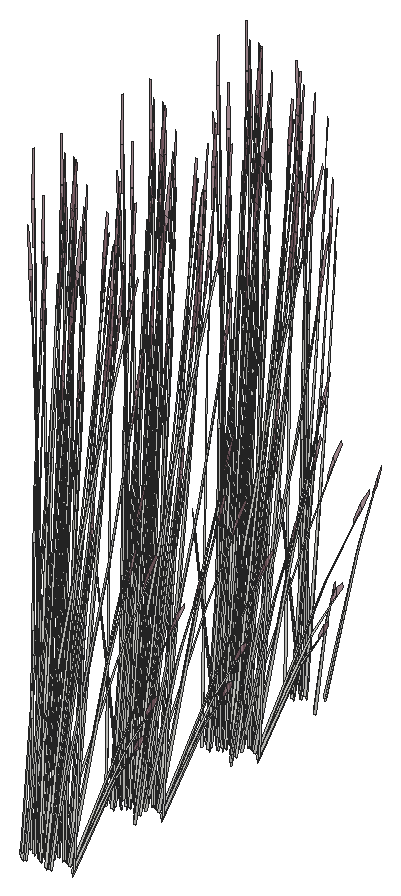
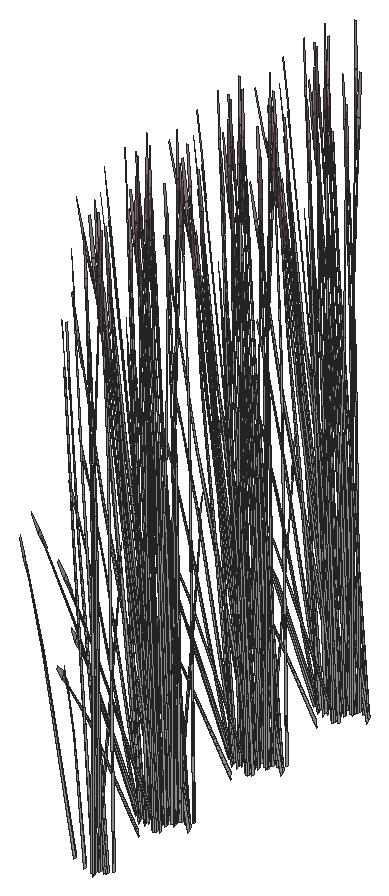
# SketchUp Ruby script. Lengths in inches.
U = 1.inch
M = Sketchup.active_model
def pt(a) = Geom::Point3d.new(a.map { |v| v * U })
def face(e, loops, mat)
  f = e.add_face(loops[0].map { |a| pt(a) })
  loops[1..].each { |l| e.add_face(l.map { |a| pt(a) }).erase! }
  f.material = f.back_material = mat if mat
  f
end
# faces: each face lists its corners as indices into pts; further lists are holes
def faces(e, pts, list, mat = nil) = list.each { |f| face(e, (f[0].is_a?(Array) ? f : [f]).map { |l| l.map { |i| pts[i] } }, mat) }
# xy, xz, yz: faces in a plane at the given z, y or x. An outline is a flat list of corners, or four numbers for a rectangle; further outlines are holes
def ring(l) = l.size == 4 ? [[l[0], l[1]], [l[2], l[1]], [l[2], l[3]], [l[0], l[3]]] : l.each_slice(2).to_a
def flat(e, list, mat, &to3) = list.each { |f| face(e, (f[0].is_a?(Array) ? f : [f]).map { |l| ring(l).map { |u, v| to3.(u, v) } }, mat) }
def xy(e, z, list, mat = nil) = flat(e, list, mat) { |x, y| [x, y, z] }
def xz(e, y, list, mat = nil) = flat(e, list, mat) { |x, z| [x, y, z] }
def yz(e, x, list, mat = nil) = flat(e, list, mat) { |y, z| [x, y, z] }
def lines(e, pts, list) = list.each { |a, b| e.add_line(pt(pts[a]), pt(pts[b])) }
# prism: a flat outline (further loops are holes) pulled along v
def prism(e, loops, v, mat = nil)
  f = face(e, loops, mat); d = Geom::Vector3d.new(v.map { |x| x * U })
  f.pushpull(f.normal.samedirection?(d) ? d.length : -d.length)
end
def box(e, o, s, mat = nil) = prism(e, [[o, [o[0] + s[0], o[1], o[2]], [o[0] + s[0], o[1] + s[1], o[2]], [o[0], o[1] + s[1], o[2]]]], [0, 0, s[2]], mat)
def at(x, y, z, deg = 0) = Geom::Transformation.translation(pt([x, y, z])) * Geom::Transformation.rotation(ORIGIN, Z_AXIS, deg.degrees)
def axes(o, x, y, z) = Geom::Transformation.new([*x, 0, *y, 0, *z, 0, *pt(o).to_a, 1])
def part(name) = M.definitions.add(name)
# library, detail: a bought-in or finely detailed component or shape, given as its bounding box
def library(name, o, s) = part(name).tap { |d| box(d.entities, o, s) }
def detail(e, o, s) = box(e.add_group.entities, o, s)
def put(e, d, t, mat = nil) = e.add_instance(d, t).tap { |i| i.material = mat if mat }
def group(e, t, mat = nil) = e.add_group.tap { |g| g.transformation = t; g.material = mat if mat }.entities
root = M.entities
M.materials.add("LightPink_Translucent").color = [144, 107, 117]
M.materials["LightPink_Translucent"].alpha = 0.75
c1 = part("blade")
p = [[2.15,0.21,22],[0,0.17,0],[0.09,0.45,0],[2.18,0.31,22],[2.29,0.31,22],[0.38,0.45,0],
  [2.48,0.24,33],[2.49,0.24,33],[2.48,0.22,33]]
faces(c1.entities,p,[[0,1,2,3],[4,5,2,3],[6,3,4,7],[8,0,3,6]])
c2 = part("seeds")
p = [[0.3,-0.1,1.38],[-0.01,-0.03,1.59],[-0.01,-0.03,0.03],[0.14,-0.07,-0.07],[0.29,-0.03,3],[0.15,0.01,3.11]]
faces(c2.entities,p,[[0,1,2,3],[1,0,4,5]],"LightPink_Translucent")
c3 = part("blade with seeds")
put(c3.entities,c1,at(0,0,0))
put(c3.entities,c2,axes([2.4,0.25,30.99],[1.5799,-0.05474,1.17369],[-0.12525,1.92788,0.29478],[-0.07173,-0.02425,1.56792]))
put(root,c3,axes([333.54,335.91,50.36],[-0.05884,-0.44587,-0.25709],[0.6128,-0.02696,-0.44182],[0.10791,-0.05939,1.41118]))
put(root,c3,axes([333.46,334.92,49.79],[0.47106,0.09668,-0.27372],[-0.11861,0.34048,0.27372],[0.09497,-0.03926,1.22797]))
put(root,c3,axes([333.62,336.26,50.15],[0.56891,0.18939,0.21263],[-0.2738,0.39352,0.44182],[0,-0.09071,1.41855]))
put(root,c3,axes([333.44,335.99,50.4],[-0.54829,0.02412,0.39531],[-0.04958,-0.40041,-0.19025],[0.09816,-0.04058,1.26923]))
put(root,c3,axes([335.24,334.92,50.1],[0.31568,-0.39156,0],[0.52815,0.21836,-0.456],[0.12029,0.04973,1.44655]))
put(root,c3,axes([336.49,336.47,49.75],[-0.3252,0.04689,1.25103],[-0.05176,-0.37326,0.07161],[0.22777,-0.0565,0.71188]))
put(root,c3,axes([337.08,336.14,50],[-0.31304,-0.24986,-0.05733],[0.34284,-0.22894,-0.25992],[0.09714,-0.01612,0.85731]))
put(root,c3,axes([334.21,336.17,49.95],[0,-0.45213,0],[0.63136,0,0],[0,0,1.58567]))
put(root,c3,axes([334.97,335.13,50.19],[-0.47255,-0.19538,0.43871],[0.28245,-0.35034,0],[0.10763,0.0445,1.3917]))
put(root,c3,axes([333.91,335.89,50.09],[-0.41865,0.35461,0.40429],[-0.49737,-0.31303,0.15865],[0.10093,-0.03539,1.40366]))
put(root,c3,axes([333.18,335.31,50.1875],[-0.14586,0.38834,0.15589],[-0.53375,-0.1099,0.31002],[0.0922,-0.00189,1.41735]))
put(root,c3,axes([332.96,335.62,49.41],[-0.49699,0.15644,1.13921],[-0.15819,-0.44887,0.44265],[0.30518,0.00747,1.29573]))
put(root,c3,axes([334.29,335.74,50.3125],[0.09741,-0.34873,0.12794],[0.4759,0.06053,-0.36534],[0.08661,0.03581,1.11991]))
put(root,c3,axes([336.84,336.23,49.32],[-0.02639,-0.05932,1.55816],[0.18302,-0.34702,-0.23804],[0.18462,-0.00499,0.26541]))
put(root,c3,axes([334.09,335.83,50.4],[-0.30332,-0.32798,0.39531],[0.45944,-0.23096,-0.19025],[0.09816,0.04058,1.26923]))
put(root,c3,axes([334.25,335.85,50.36],[0.50979,-0.25942,-0.25709],[0.339,0.36656,-0.44182],[0.12578,0.03723,1.41118]))
put(root,c3,axes([335.53,335.16,49.78],[0.47255,0.19538,-0.43871],[-0.28245,0.35034,0],[0.10763,0.0445,1.3917]))
put(root,c3,axes([334.63,336.28,49.95],[0.56491,0,0],[0,0.40454,0],[0,0,1.5764]))
put(root,c3,axes([334.79,335.33,50.1875],[-0.54257,0.10371,0.15589],[-0.13397,-0.38597,0.31002],[0.04839,0.05624,1.41735]))
put(root,c3,axes([335.4,335.31,49.79],[0.11861,0.34048,-0.27372],[-0.47106,0.09668,0.27372],[0.09497,0.03926,1.22797]))
put(root,c3,axes([334.45,336.07,50.1],[-0.63817,-0.08233,0.43472],[0.12987,-0.46497,0.17059],[0.09326,0.0449,1.50931]))
put(root,c3,axes([334.56,337.17,49.93],[0.53009,-0.13258,-0.16963],[0.18627,0.38191,0.00007],[0.05851,-0.01465,1.53656]))
put(root,c3,axes([334.62,336.45,49.96],[0.35245,0.2524,0],[-0.35245,0.2524,0],[0,0,1.49564]))
put(root,c3,axes([335.58,336.34,50.1875],[-0.39671,-0.28463,0.15589],[0.39978,-0.27607,0.31002],[-0.04381,0.05813,1.41735]))
put(root,c3,axes([334.84,335.91,49.82],[0.52523,0.06406,-0.55095],[-0.11084,0.39517,-0.1446],[0.15674,0.04788,1.21613]))
put(root,c3,axes([334.62,336.15,50.4],[0.24498,-0.3521,0.39531],[0.50902,0.16945,-0.19025],[0,0.08116,1.26923]))
put(root,c3,axes([334.52,336.35,50.03],[0,0.45191,-0.04981],[-0.63136,0,0],[0,0.0142,1.58489]))
put(root,c3,axes([334.57,336.03,49.95],[0.30332,0.32798,-0.39531],[-0.45944,0.23096,0.19025],[0.09816,0.04058,1.26923]))
put(root,c3,axes([335.9,336.35,50.19],[0,-0.39075,0.43871],[0.56491,0,0],[0,0.089,1.3917]))
put(root,c3,axes([334.83,336.23,50.3125],[0.47043,-0.11396,0.12794],[0.16474,0.32541,-0.36534],[0,0.07162,1.11991]))
put(root,c3,axes([336.58,337.03,50.29],[-0.1216,-0.0961,1.26356],[0.15822,-0.31792,-0.27174],[0.24603,0.04307,0.54024]))
put(root,c3,axes([334.4,337.375,49.95],[0.50902,0.17543,0],[-0.24498,0.36452,0],[0,0,1.54589]))
put(root,c3,axes([334.22,337.23,50.02],[0.21952,0.44891,-0.05313],[-0.62724,0.1573,0],[0.00767,0.01568,1.52132]))
put(root,c3,axes([336.29,336.42,50.1],[0.63136,0,0],[0,0.43672,-0.456],[0,0.09947,1.44655]))
put(root,c3,axes([336.03,336.64,49.94],[-0.63105,-0.00312,-0.04397],[0,-0.43672,0.44129],[-0.01983,0.09942,1.3992]))
put(root,c3,axes([334.67,336.26,50.36],[0.56863,0.18645,-0.25709],[-0.2738,0.39352,-0.44182],[0.01787,0.09662,1.41118]))
put(root,c3,axes([335.9,336.7,49.79],[-0.35245,0.2438,-0.27372],[-0.35245,-0.2438,0.27372],[0,0.07853,1.22797]))
put(root,c3,axes([336.15,336.71,49.78],[0,0.39075,-0.43871],[-0.56491,0,0],[0,0.089,1.3917]))
put(root,c3,axes([335.51,337.94,49.32],[0.03679,-0.05641,1.55816],[0.46313,-0.16615,-0.23804],[0.14041,0.08599,0.26541]))
put(root,c3,axes([334.9,336.66,49.85],[0.18514,0.35777,-0.61156],[-0.53331,0.12885,-0.16051],[0.02046,0.12115,1.3499]))
put(root,c3,axes([335.47,338.03,50.36],[-0.32378,-0.01225,0.92831],[0.21383,-0.26028,0.51254],[0.12791,0.09247,0.72818]))
put(root,c3,axes([334.42,337.4,50.29],[0.00891,-0.12953,1.26356],[0.4258,-0.14469,-0.27174],[0.13144,0.15503,0.54024]))
put(root,c3,axes([334.77,344.44,50.29],[-0.14352,0.07909,1.26356],[-0.42983,-0.13843,-0.27174],[0.07968,-0.17216,0.54024]))
put(root,c3,axes([335.77,344.6875,49.32],[-0.07557,-0.03078,1.55816],[-0.19412,-0.34391,-0.23804],[0.13095,-0.09333,0.26541]))
put(root,c3,axes([332.92,344.76,50.1],[-0.31568,-0.39156,0],[0.52815,-0.21836,-0.456],[0.12029,-0.04973,1.44655]))
put(root,c3,axes([333.35,344.7,49.78],[0.47255,-0.19538,-0.43871],[0.28245,0.35034,0],[0.10763,-0.0445,1.3917]))
put(root,c3,axes([336.15,345.375,50.29],[-0.18038,-0.01157,1.26356],[-0.18479,-0.31048,-0.27174],[0.22159,-0.08783,0.54024]))
put(root,c3,axes([333.91,345.5,49.82],[0.34009,-0.2937,-0.55095],[0.42248,0.26632,-0.1446],[0.13628,-0.07327,1.21613]))
put(root,c3,axes([333.54,345.84,50.36],[-0.05884,-0.44587,-0.25709],[0.6128,-0.02696,-0.44182],[0.10791,-0.05939,1.41118]))
put(root,c3,axes([333.46,344.86,49.79],[0.47106,0.09668,-0.27372],[-0.11861,0.34048,0.27372],[0.09497,-0.03926,1.22797]))
put(root,c3,axes([333.62,346.19,50.15],[0.56891,0.18939,0.21263],[-0.2738,0.39352,0.44182],[0,-0.09071,1.41855]))
put(root,c3,axes([333.44,345.93,50.4],[-0.54829,0.02412,0.39531],[-0.04958,-0.40041,-0.19025],[0.09816,-0.04058,1.26923]))
put(root,c3,axes([335.24,344.86,50.1],[0.31568,-0.39156,0],[0.52815,0.21836,-0.456],[0.12029,0.04973,1.44655]))
put(root,c3,axes([336.49,346.41,49.75],[-0.3252,0.04689,1.25103],[-0.05176,-0.37326,0.07161],[0.22777,-0.0565,0.71188]))
put(root,c3,axes([337.08,346.08,50],[-0.31304,-0.24986,-0.05733],[0.34284,-0.22894,-0.25992],[0.09714,-0.01612,0.85731]))
put(root,c3,axes([334.21,346.11,49.95],[0,-0.45213,0],[0.63136,0,0],[0,0,1.58567]))
put(root,c3,axes([334.97,345.06,50.19],[-0.47255,-0.19538,0.43871],[0.28245,-0.35034,0],[0.10763,0.0445,1.3917]))
put(root,c3,axes([333.91,345.82,50.09],[-0.41865,0.35461,0.40429],[-0.49737,-0.31303,0.15865],[0.10093,-0.03539,1.40366]))
put(root,c3,axes([333.18,345.24,50.1875],[-0.14586,0.38834,0.15589],[-0.53375,-0.1099,0.31002],[0.0922,-0.00189,1.41735]))
put(root,c3,axes([332.96,345.55,49.41],[-0.49699,0.15644,1.13921],[-0.15819,-0.44887,0.44265],[0.30518,0.00747,1.29573]))
put(root,c3,axes([334.29,345.67,50.3125],[0.09741,-0.34873,0.12794],[0.4759,0.06053,-0.36534],[0.08661,0.03581,1.11991]))
put(root,c3,axes([336.84,346.16,49.32],[-0.02639,-0.05932,1.55816],[0.18302,-0.34702,-0.23804],[0.18462,-0.00499,0.26541]))
put(root,c3,axes([334.09,345.76,50.4],[-0.30332,-0.32798,0.39531],[0.45944,-0.23096,-0.19025],[0.09816,0.04058,1.26923]))
put(root,c3,axes([334.25,345.79,50.36],[0.50979,-0.25942,-0.25709],[0.339,0.36656,-0.44182],[0.12578,0.03723,1.41118]))
put(root,c3,axes([335.53,345.1,49.78],[0.47255,0.19538,-0.43871],[-0.28245,0.35034,0],[0.10763,0.0445,1.3917]))
put(root,c3,axes([334.63,346.21,49.95],[0.56491,0,0],[0,0.40454,0],[0,0,1.5764]))
put(root,c3,axes([334.79,345.26,50.1875],[-0.54257,0.10371,0.15589],[-0.13397,-0.38597,0.31002],[0.04839,0.05624,1.41735]))
put(root,c3,axes([335.4,345.24,49.79],[0.11861,0.34048,-0.27372],[-0.47106,0.09668,0.27372],[0.09497,0.03926,1.22797]))
put(root,c3,axes([334.45,346,50.1],[-0.63817,-0.08233,0.43472],[0.12987,-0.46497,0.17059],[0.09326,0.0449,1.50931]))
put(root,c3,axes([334.56,347.11,49.93],[0.53009,-0.13258,-0.16963],[0.18627,0.38191,0.00007],[0.05851,-0.01465,1.53656]))
put(root,c3,axes([334.62,346.38,49.96],[0.35245,0.2524,0],[-0.35245,0.2524,0],[0,0,1.49564]))
put(root,c3,axes([335.58,346.27,50.1875],[-0.39671,-0.28463,0.15589],[0.39978,-0.27607,0.31002],[-0.04381,0.05813,1.41735]))
put(root,c3,axes([334.84,345.84,49.82],[0.52523,0.06406,-0.55095],[-0.11084,0.39517,-0.1446],[0.15674,0.04788,1.21613]))
put(root,c3,axes([334.62,346.09,50.4],[0.24498,-0.3521,0.39531],[0.50902,0.16945,-0.19025],[0,0.08116,1.26923]))
put(root,c3,axes([334.52,346.29,50.03],[0,0.45191,-0.04981],[-0.63136,0,0],[0,0.0142,1.58489]))
put(root,c3,axes([334.57,345.97,49.95],[0.30332,0.32798,-0.39531],[-0.45944,0.23096,0.19025],[0.09816,0.04058,1.26923]))
put(root,c3,axes([335.9,346.28,50.19],[0,-0.39075,0.43871],[0.56491,0,0],[0,0.089,1.3917]))
put(root,c3,axes([334.83,346.17,50.3125],[0.47043,-0.11396,0.12794],[0.16474,0.32541,-0.36534],[0,0.07162,1.11991]))
put(root,c3,axes([336.58,346.96,50.29],[-0.1216,-0.0961,1.26356],[0.15822,-0.31792,-0.27174],[0.24603,0.04307,0.54024]))
put(root,c3,axes([334.4,347.3125,49.95],[0.50902,0.17543,0],[-0.24498,0.36452,0],[0,0,1.54589]))
put(root,c3,axes([334.22,347.16,50.02],[0.21952,0.44891,-0.05313],[-0.62724,0.1573,0],[0.00767,0.01568,1.52132]))
put(root,c3,axes([336.29,346.35,50.1],[0.63136,0,0],[0,0.43672,-0.456],[0,0.09947,1.44655]))
put(root,c3,axes([336.03,346.58,49.94],[-0.63105,-0.00312,-0.04397],[0,-0.43672,0.44129],[-0.01983,0.09942,1.3992]))
put(root,c3,axes([334.67,346.2,50.36],[0.56863,0.18645,-0.25709],[-0.2738,0.39352,-0.44182],[0.01787,0.09662,1.41118]))
put(root,c3,axes([335.9,346.64,49.79],[-0.35245,0.2438,-0.27372],[-0.35245,-0.2438,0.27372],[0,0.07853,1.22797]))
put(root,c3,axes([336.15,346.65,49.78],[0,0.39075,-0.43871],[-0.56491,0,0],[0,0.089,1.3917]))
put(root,c3,axes([335.51,347.875,49.32],[0.03679,-0.05641,1.55816],[0.46313,-0.16615,-0.23804],[0.14041,0.08599,0.26541]))
put(root,c3,axes([334.9,346.59,49.85],[0.18514,0.35777,-0.61156],[-0.53331,0.12885,-0.16051],[0.02046,0.12115,1.3499]))
put(root,c3,axes([335.47,347.97,50.36],[-0.32378,-0.01225,0.92831],[0.21383,-0.26028,0.51254],[0.12791,0.09247,0.72818]))
put(root,c3,axes([334.42,347.34,50.29],[0.00891,-0.12953,1.26356],[0.4258,-0.14469,-0.27174],[0.13144,0.15503,0.54024]))
put(root,c3,axes([334.77,355.17,50.29],[-0.14352,0.07909,1.26356],[-0.42983,-0.13843,-0.27174],[0.07968,-0.17216,0.54024]))
put(root,c3,axes([335.77,355.41,49.32],[-0.07557,-0.03078,1.55816],[-0.19412,-0.34391,-0.23804],[0.13095,-0.09333,0.26541]))
put(root,c3,axes([332.92,355.48,50.1],[-0.31568,-0.39156,0],[0.52815,-0.21836,-0.456],[0.12029,-0.04973,1.44655]))
put(root,c3,axes([333.35,355.42,49.78],[0.47255,-0.19538,-0.43871],[0.28245,0.35034,0],[0.10763,-0.0445,1.3917]))
put(root,c3,axes([336.15,356.1,50.29],[-0.18038,-0.01157,1.26356],[-0.18479,-0.31048,-0.27174],[0.22159,-0.08783,0.54024]))
put(root,c3,axes([333.91,356.22,49.82],[0.34009,-0.2937,-0.55095],[0.42248,0.26632,-0.1446],[0.13628,-0.07327,1.21613]))
put(root,c3,axes([333.54,356.56,50.36],[-0.05884,-0.44587,-0.25709],[0.6128,-0.02696,-0.44182],[0.10791,-0.05939,1.41118]))
put(root,c3,axes([333.46,355.58,49.79],[0.47106,0.09668,-0.27372],[-0.11861,0.34048,0.27372],[0.09497,-0.03926,1.22797]))
put(root,c3,axes([333.62,356.91,50.15],[0.56891,0.18939,0.21263],[-0.2738,0.39352,0.44182],[0,-0.09071,1.41855]))
put(root,c3,axes([333.44,356.65,50.4],[-0.54829,0.02412,0.39531],[-0.04958,-0.40041,-0.19025],[0.09816,-0.04058,1.26923]))
put(root,c3,axes([335.24,355.58,50.1],[0.31568,-0.39156,0],[0.52815,0.21836,-0.456],[0.12029,0.04973,1.44655]))
put(root,c3,axes([336.49,357.13,49.75],[-0.3252,0.04689,1.25103],[-0.05176,-0.37326,0.07161],[0.22777,-0.0565,0.71188]))
put(root,c3,axes([337.08,356.8,50],[-0.31304,-0.24986,-0.05733],[0.34284,-0.22894,-0.25992],[0.09714,-0.01612,0.85731]))
put(root,c3,axes([334.21,356.83,49.95],[0,-0.45213,0],[0.63136,0,0],[0,0,1.58567]))
put(root,c3,axes([334.97,355.79,50.19],[-0.47255,-0.19538,0.43871],[0.28245,-0.35034,0],[0.10763,0.0445,1.3917]))
put(root,c3,axes([333.91,356.55,50.09],[-0.41865,0.35461,0.40429],[-0.49737,-0.31303,0.15865],[0.10093,-0.03539,1.40366]))
put(root,c3,axes([333.18,355.96,50.1875],[-0.14586,0.38834,0.15589],[-0.53375,-0.1099,0.31002],[0.0922,-0.00189,1.41735]))
put(root,c3,axes([332.96,356.28,49.41],[-0.49699,0.15644,1.13921],[-0.15819,-0.44887,0.44265],[0.30518,0.00747,1.29573]))
put(root,c3,axes([334.29,356.39,50.3125],[0.09741,-0.34873,0.12794],[0.4759,0.06053,-0.36534],[0.08661,0.03581,1.11991]))
put(root,c3,axes([336.84,356.89,49.32],[-0.02639,-0.05932,1.55816],[0.18302,-0.34702,-0.23804],[0.18462,-0.00499,0.26541]))
put(root,c3,axes([334.09,356.49,50.4],[-0.30332,-0.32798,0.39531],[0.45944,-0.23096,-0.19025],[0.09816,0.04058,1.26923]))
put(root,c3,axes([334.25,356.51,50.36],[0.50979,-0.25942,-0.25709],[0.339,0.36656,-0.44182],[0.12578,0.03723,1.41118]))
put(root,c3,axes([335.53,355.82,49.78],[0.47255,0.19538,-0.43871],[-0.28245,0.35034,0],[0.10763,0.0445,1.3917]))
put(root,c3,axes([334.63,356.93,49.95],[0.56491,0,0],[0,0.40454,0],[0,0,1.5764]))
put(root,c3,axes([334.79,355.98,50.1875],[-0.54257,0.10371,0.15589],[-0.13397,-0.38597,0.31002],[0.04839,0.05624,1.41735]))
put(root,c3,axes([335.4,355.96,49.79],[0.11861,0.34048,-0.27372],[-0.47106,0.09668,0.27372],[0.09497,0.03926,1.22797]))
put(root,c3,axes([334.45,356.73,50.1],[-0.63817,-0.08233,0.43472],[0.12987,-0.46497,0.17059],[0.09326,0.0449,1.50931]))
put(root,c3,axes([334.56,357.83,49.93],[0.53009,-0.13258,-0.16963],[0.18627,0.38191,0.00007],[0.05851,-0.01465,1.53656]))
put(root,c3,axes([334.62,357.11,49.96],[0.35245,0.2524,0],[-0.35245,0.2524,0],[0,0,1.49564]))
put(root,c3,axes([335.58,357,50.1875],[-0.39671,-0.28463,0.15589],[0.39978,-0.27607,0.31002],[-0.04381,0.05813,1.41735]))
put(root,c3,axes([334.84,356.57,49.82],[0.52523,0.06406,-0.55095],[-0.11084,0.39517,-0.1446],[0.15674,0.04788,1.21613]))
put(root,c3,axes([334.62,356.8125,50.4],[0.24498,-0.3521,0.39531],[0.50902,0.16945,-0.19025],[0,0.08116,1.26923]))
put(root,c3,axes([334.52,357.01,50.03],[0,0.45191,-0.04981],[-0.63136,0,0],[0,0.0142,1.58489]))
put(root,c3,axes([334.57,356.69,49.95],[0.30332,0.32798,-0.39531],[-0.45944,0.23096,0.19025],[0.09816,0.04058,1.26923]))
put(root,c3,axes([335.9,357.01,50.19],[0,-0.39075,0.43871],[0.56491,0,0],[0,0.089,1.3917]))
put(root,c3,axes([334.83,356.89,50.3125],[0.47043,-0.11396,0.12794],[0.16474,0.32541,-0.36534],[0,0.07162,1.11991]))
put(root,c3,axes([336.58,357.68,50.29],[-0.1216,-0.0961,1.26356],[0.15822,-0.31792,-0.27174],[0.24603,0.04307,0.54024]))
put(root,c3,axes([334.4,358.03,49.95],[0.50902,0.17543,0],[-0.24498,0.36452,0],[0,0,1.54589]))
put(root,c3,axes([334.22,357.89,50.02],[0.21952,0.44891,-0.05313],[-0.62724,0.1573,0],[0.00767,0.01568,1.52132]))
put(root,c3,axes([336.29,357.07,50.1],[0.63136,0,0],[0,0.43672,-0.456],[0,0.09947,1.44655]))
put(root,c3,axes([336.03,357.3,49.94],[-0.63105,-0.00312,-0.04397],[0,-0.43672,0.44129],[-0.01983,0.09942,1.3992]))
put(root,c3,axes([334.67,356.92,50.36],[0.56863,0.18645,-0.25709],[-0.2738,0.39352,-0.44182],[0.01787,0.09662,1.41118]))
put(root,c3,axes([335.9,357.36,49.79],[-0.35245,0.2438,-0.27372],[-0.35245,-0.2438,0.27372],[0,0.07853,1.22797]))
put(root,c3,axes([336.15,357.37,49.78],[0,0.39075,-0.43871],[-0.56491,0,0],[0,0.089,1.3917]))
put(root,c3,axes([335.51,358.6,49.32],[0.03679,-0.05641,1.55816],[0.46313,-0.16615,-0.23804],[0.14041,0.08599,0.26541]))
put(root,c3,axes([334.9,357.32,49.85],[0.18514,0.35777,-0.61156],[-0.53331,0.12885,-0.16051],[0.02046,0.12115,1.3499]))
put(root,c3,axes([335.47,358.69,50.36],[-0.32378,-0.01225,0.92831],[0.21383,-0.26028,0.51254],[0.12791,0.09247,0.72818]))
put(root,c3,axes([334.42,358.0625,50.29],[0.00891,-0.12953,1.26356],[0.4258,-0.14469,-0.27174],[0.13144,0.15503,0.54024]))
put(root,c3,axes([334.77,364.49,50.29],[-0.14352,0.07909,1.26356],[-0.42983,-0.13843,-0.27174],[0.07968,-0.17216,0.54024]))
put(root,c3,axes([335.77,364.74,49.32],[-0.07557,-0.03078,1.55816],[-0.19412,-0.34391,-0.23804],[0.13095,-0.09333,0.26541]))
put(root,c3,axes([332.92,364.81,50.1],[-0.31568,-0.39156,0],[0.52815,-0.21836,-0.456],[0.12029,-0.04973,1.44655]))
put(root,c3,axes([333.35,364.75,49.78],[0.47255,-0.19538,-0.43871],[0.28245,0.35034,0],[0.10763,-0.0445,1.3917]))
put(root,c3,axes([336.15,365.42,50.29],[-0.18038,-0.01157,1.26356],[-0.18479,-0.31048,-0.27174],[0.22159,-0.08783,0.54024]))
put(root,c3,axes([333.91,365.55,49.82],[0.34009,-0.2937,-0.55095],[0.42248,0.26632,-0.1446],[0.13628,-0.07327,1.21613]))
put(root,c3,axes([333.54,365.89,50.36],[-0.05884,-0.44587,-0.25709],[0.6128,-0.02696,-0.44182],[0.10791,-0.05939,1.41118]))
put(root,c3,axes([333.46,364.9,49.79],[0.47106,0.09668,-0.27372],[-0.11861,0.34048,0.27372],[0.09497,-0.03926,1.22797]))
put(root,c3,axes([333.62,366.24,50.15],[0.56891,0.18939,0.21263],[-0.2738,0.39352,0.44182],[0,-0.09071,1.41855]))
put(root,c3,axes([333.44,365.98,50.4],[-0.54829,0.02412,0.39531],[-0.04958,-0.40041,-0.19025],[0.09816,-0.04058,1.26923]))
